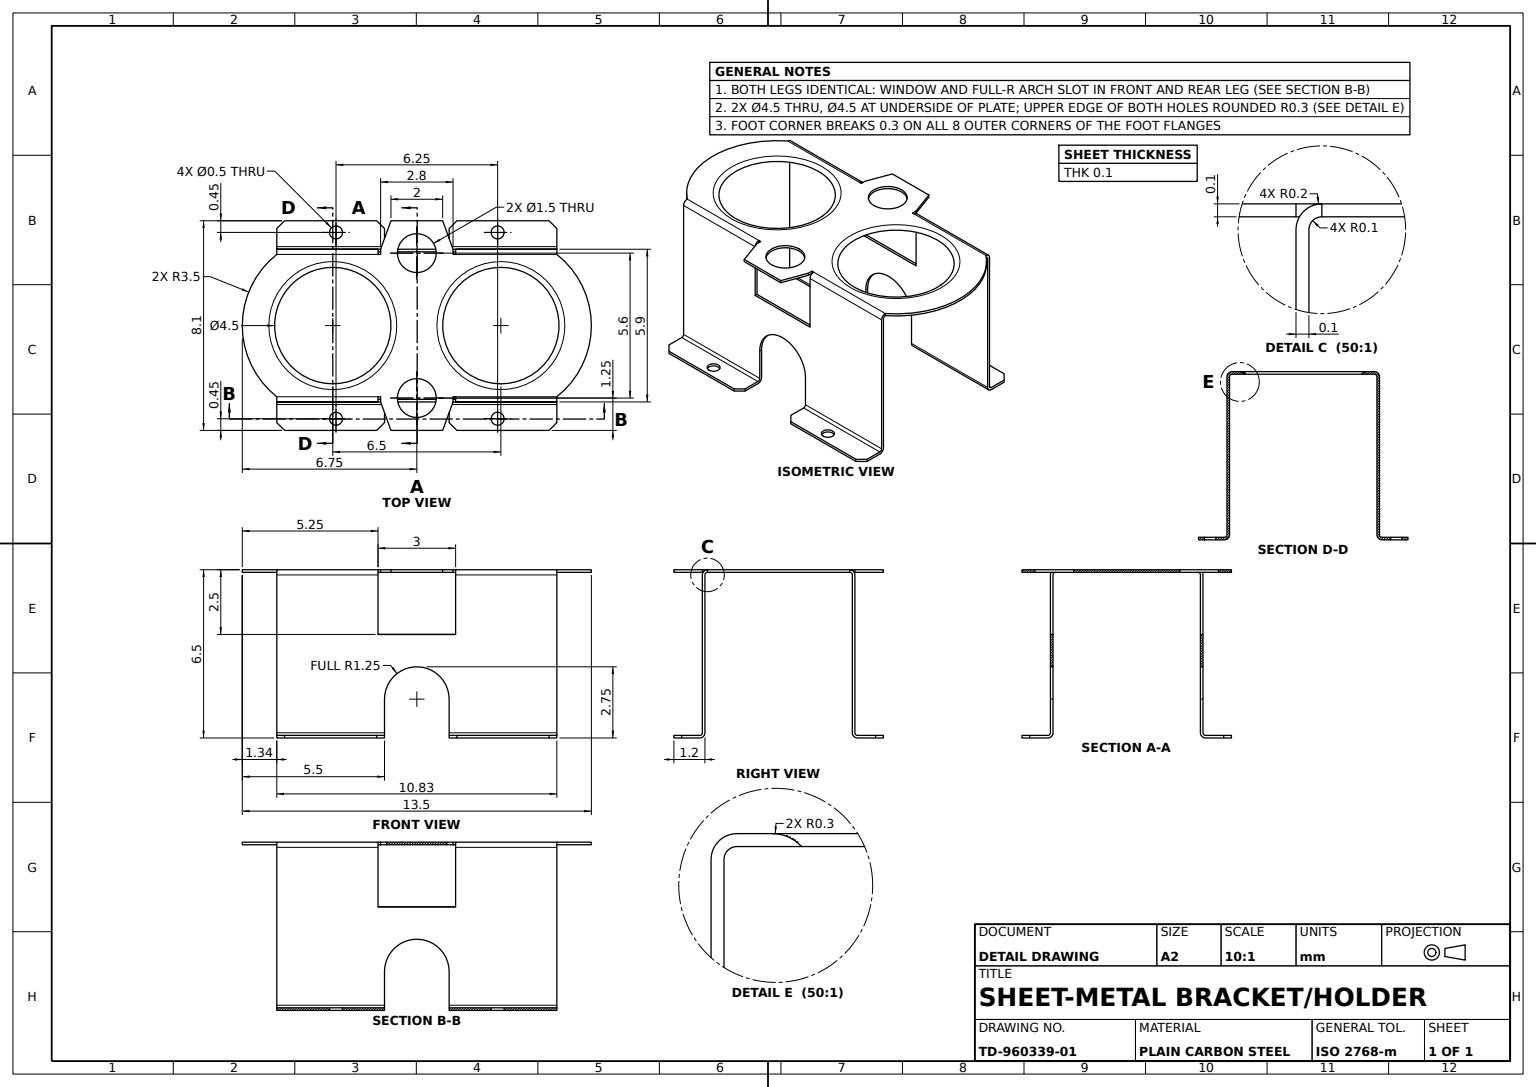
solid
v1 (-3.250103,0,-2.05)
v2 (-3.250103,0,-3.55)
e1 v1 v2 CIRCLE(AX(P(-3.250103,0,-2.8),D(0,-1,0),D(0,0,-1)),0.75)
v3 (-3.250103,-0.1,-2.05)
e2 v3 v1 LINE
v4 (-3.250103,-0.1,-3.55)
e3 v3 v4 CIRCLE(AX(P(-3.250103,-0.1,-2.8),D(0,-1,0),D(0,0,-1)),0.75)
e4 v4 v2 LINE
face CYL(AX(P(-3.250103,-0.1,-2.8),D(0,1,0),D(0,0,1)),0.75) rev [-e1 -e2 e3 e4]
v5 (2.164897,-6.3,-2.85)
v6 (2.164897,-6.5,-3.05)
e5 v5 v6 CIRCLE(AX(P(2.164897,-6.3,-3.05),D(1,0,0),D(0,0,1)),0.2)
v7 (-2.000103,-6.3,-2.85)
e6 v7 v5 LINE
v8 (-2.000103,-6.5,-3.05)
e7 v7 v8 CIRCLE(AX(P(-2.000103,-6.3,-3.05),D(1,0,0),D(0,-1,0)),0.2)
e8 v8 v6 LINE
face CYL(AX(P(-8.665103,-6.3,-3.05),D(-1,0,0),D(0,-1,0)),0.2) [-e5 -e6 e7 e8]
v9 (-1.750103,-0.2,2.85)
v10 (-1.750103,-0.1,2.75)
e9 v9 v10 CIRCLE(AX(P(-1.750103,-0.2,2.75),D(-1,0,0),D(0,0,-1)),0.1)
v11 (2.164897,-0.1,2.75)
e10 v10 v11 LINE
v12 (2.164897,-0.2,2.85)
e11 v11 v12 CIRCLE(AX(P(2.164897,-0.2,2.75),D(1,0,0),D(0,0,1)),0.1)
e12 v12 v9 LINE
face CYL(AX(P(-8.665103,-0.2,2.75),D(-1,0,0),D(0,0,1)),0.1) rev [e9 e10 e11 e12]
v13 (-4.750103,-2.5,2.85)
v14 (-4.750103,-2.5,2.95)
e13 v13 v14 LINE
v15 (-1.750103,-2.5,2.95)
e14 v15 v14 LINE
v16 (-1.750103,-2.5,2.85)
e15 v16 v15 LINE
e16 v16 v13 LINE
face PLANE(AX(P(-1.750103,-2.5,2.95),D(0,-1,0),D(-1,0,0))) rev [e13 -e14 -e15 e16]
v17 (-0.125103,-6.5,3.85)
v18 (-0.125103,-6.4,3.85)
e17 v17 v18 LINE
v19 (-0.125103,-6.4,3.35)
e18 v19 v18 CIRCLE(AX(P(-0.125103,-6.4,3.6),D(0,-1,0),D(0,0,1)),0.25)
v20 (-0.125103,-6.5,3.35)
e19 v20 v19 LINE
e20 v20 v17 CIRCLE(AX(P(-0.125103,-6.5,3.6),D(0,-1,0),D(0,0,1)),0.25)
face CYL(AX(P(-0.125103,-6.5,3.6),D(0,1,0),D(0,0,1)),0.25) rev [e17 -e18 -e19 e20]
v21 (-1.750103,-2.5,-2.85)
v22 (-1.750103,-2.5,-2.95)
e21 v21 v22 LINE
v23 (-4.750103,-2.5,-2.95)
e22 v23 v22 LINE
v24 (-4.750103,-2.5,-2.85)
e23 v24 v23 LINE
e24 v24 v21 LINE
face PLANE(AX(P(-4.750103,-2.5,-2.95),D(0,-1,0),D(1,0,0))) rev [e21 -e22 -e23 e24]
v25 (-2.000103,-6.5,3.05)
v26 (-2.000103,-6.3,2.85)
e25 v25 v26 CIRCLE(AX(P(-2.000103,-6.3,3.05),D(1,0,0),D(0,-1,0)),0.2)
v27 (-2.000103,-6.4,3.05)
e26 v27 v25 LINE
v28 (-2.000103,-6.3,2.95)
e27 v27 v28 CIRCLE(AX(P(-2.000103,-6.3,3.05),D(1,0,0),D(0,-1,0)),0.1)
e28 v26 v28 LINE
face PLANE(AX(P(-2.000103,-5,-4.05),D(-1,0,0),D(0,-1,0))) [-e25 -e26 e27 -e28]
v29 (2.164897,-6.4,3.75)
v30 (2.164897,-6.5,3.75)
e29 v29 v30 LINE
v31 (1.864897,-6.4,4.05)
e30 v31 v29 LINE
v32 (1.864897,-6.5,4.05)
e31 v32 v31 LINE
e32 v30 v32 LINE
face PLANE(AX(P(1.864897,-6.5,4.05),D(-0.707106781,0,-0.707106781),D(0,1,0))) rev [-e29 -e30 -e31 -e32]
v33 (-1.750103,-0.2,-2.85)
v34 (2.164897,-0.2,-2.85)
e33 v33 v34 LINE
v35 (2.164897,-0.1,-2.75)
e34 v34 v35 CIRCLE(AX(P(2.164897,-0.2,-2.75),D(1,0,0),D(0,0,-1)),0.1)
v36 (-1.750103,-0.1,-2.75)
e35 v35 v36 LINE
e36 v36 v33 CIRCLE(AX(P(-1.750103,-0.2,-2.75),D(-1,0,0),D(0,0,-1)),0.1)
face CYL(AX(P(2.164897,-0.2,-2.75),D(1,0,0),D(0,0,-1)),0.1) rev [e33 e34 e35 e36]
v37 (-1.850103,-0.1,-2.75)
v38 (-1.850103,0,-2.75)
e37 v37 v38 LINE
v39 (-1.750103,0,-2.75)
e38 v39 v38 LINE
e39 v36 v39 LINE
e40 v36 v37 LINE
face PLANE(AX(P(-1.750103,0,-2.75),D(0,0,1),D(-1,0,0))) rev [e37 -e38 -e39 e40]
v40 (-4.750103,-0.1,2.75)
v41 (-4.750103,-0.2,2.85)
e41 v40 v41 CIRCLE(AX(P(-4.750103,-0.2,2.75),D(1,0,0),D(0,0,1)),0.1)
v42 (-4.750103,0,2.75)
e42 v40 v42 LINE
v43 (-4.750103,-0.2,2.95)
e43 v42 v43 CIRCLE(AX(P(-4.750103,-0.2,2.75),D(1,0,0),D(0,0,1)),0.2)
e44 v14 v43 LINE
e45 v13 v41 LINE
face PLANE(AX(P(-4.750103,-0.2,2.75),D(-1,0,0),D(0,0,1))) rev [-e41 e42 e43 -e44 -e13 e45]
v44 (-8.665103,-6.5,3.75)
v45 (-8.665103,-6.4,3.75)
e46 v44 v45 LINE
v46 (-8.665103,-6.4,3.05)
e47 v45 v46 LINE
v47 (-8.665103,-6.5,3.05)
e48 v46 v47 LINE
e49 v44 v47 LINE
face PLANE(AX(P(-8.665103,-6.5,2.95),D(1,0,0),D(0,0,-1))) rev [e46 e47 e48 -e49]
v48 (-8.665103,-6.5,-3.05)
v49 (-4.500103,-6.5,-3.05)
e50 v48 v49 LINE
v50 (-4.500103,-6.3,-2.85)
e51 v49 v50 CIRCLE(AX(P(-4.500103,-6.3,-3.05),D(-1,0,0),D(0,1,0)),0.2)
v51 (-8.665103,-6.3,-2.85)
e52 v51 v50 LINE
e53 v48 v51 CIRCLE(AX(P(-8.665103,-6.3,-3.05),D(-1,0,0),D(0,0,1)),0.2)
face CYL(AX(P(-8.665103,-6.3,-3.05),D(-1,0,0),D(0,-1,0)),0.2) [e50 e51 -e52 -e53]
v52 (-4.250103,0,4.05)
v53 (-2.250103,0,4.05)
e54 v52 v53 LINE
v54 (-4.250103,-0.1,4.05)
e55 v54 v52 LINE
v55 (-2.250103,-0.1,4.05)
e56 v54 v55 LINE
e57 v55 v53 LINE
face PLANE(AX(P(-2.250103,-0.1,4.05),D(0,0,1),D(1,0,0))) [-e54 -e55 e56 e57]
v56 (-8.665103,-0.2,2.95)
v57 (-8.665103,-6.3,2.95)
e58 v56 v57 LINE
v58 (-4.500103,-6.3,2.95)
e59 v58 v57 LINE
v59 (-4.500103,-5,2.95)
e60 v59 v58 LINE
v60 (-2.000103,-5,2.95)
e61 v60 v59 CIRCLE(AX(P(-3.250103,-5,2.95),D(0,0,1),D(0,1,0)),1.25)
e62 v28 v60 LINE
v61 (2.164897,-6.3,2.95)
e63 v61 v28 LINE
v62 (2.164897,-0.2,2.95)
e64 v61 v62 LINE
v63 (-1.750103,-0.2,2.95)
e65 v63 v62 LINE
e66 v15 v63 LINE
e67 v56 v43 LINE
face PLANE(AX(P(0,0,2.95),D(0,0,-1),D(0,1,0))) rev [e58 -e59 -e60 -e61 -e62 -e63 e64 -e65 -e66 e14 e44 -e67]
v64 (-2.000103,-5,2.85)
e68 v64 v60 LINE
e69 v26 v64 LINE
face PLANE(AX(P(-2.000103,-5,-4.05),D(-1,0,0),D(0,-1,0))) [-e68 -e69 e28 e62]
v65 (-4.500103,-6.4,3.05)
e70 v58 v65 CIRCLE(AX(P(-4.500103,-6.3,3.05),D(-1,0,0),D(0,1,0)),0.1)
e71 v57 v46 CIRCLE(AX(P(-8.665103,-6.3,3.05),D(-1,0,0),D(0,0,-1)),0.1)
e72 v46 v65 LINE
face CYL(AX(P(2.164897,-6.3,3.05),D(1,0,0),D(0,-1,0)),0.1) rev [-e70 e59 e71 e72]
v66 (2.164897,-6.4,3.05)
e73 v66 v29 LINE
v67 (2.164897,-6.5,3.05)
e74 v67 v30 LINE
e75 v66 v67 LINE
face PLANE(AX(P(2.164897,-6.5,4.05),D(-1,0,0),D(0,0,1))) rev [e73 e29 -e74 -e75]
v68 (-2.000103,-6.4,-3.05)
e76 v8 v68 LINE
v69 (-2.000103,-6.4,-3.75)
e77 v69 v68 LINE
v70 (-2.000103,-6.5,-3.75)
e78 v69 v70 LINE
e79 v70 v8 LINE
face PLANE(AX(P(-2.000103,-5,-4.05),D(-1,0,0),D(0,-1,0))) [e76 -e77 e78 e79]
e80 v9 v16 LINE
v71 (-1.750103,0,2.75)
e81 v63 v71 CIRCLE(AX(P(-1.750103,-0.2,2.75),D(-1,0,0),D(0,0,1)),0.2)
e82 v10 v71 LINE
face PLANE(AX(P(-1.750103,-0.2,2.75),D(1,0,0),D(0,0,-1))) rev [e80 e15 e66 e81 -e82 -e9]
v72 (-4.500103,-6.4,-3.75)
v73 (-4.800103,-6.4,-4.05)
e83 v72 v73 LINE
v74 (-4.500103,-6.5,-3.75)
e84 v74 v72 LINE
v75 (-4.800103,-6.5,-4.05)
e85 v75 v74 LINE
e86 v73 v75 LINE
face PLANE(AX(P(-4.500103,-6.5,-3.75),D(0.707106781,0,-0.707106781),D(0,-1,0))) [-e83 -e84 -e85 -e86]
v76 (-1.850103,-0.1,-2.95)
v77 (-1.850103,0,-2.95)
e87 v76 v77 LINE
e88 v77 v38 LINE
e89 v76 v37 LINE
face PLANE(AX(P(-1.850103,-0.1,-2.95),D(-1,0,0),D(0,0,1))) rev [e87 e88 -e37 -e89]
v78 (-6.375103,-6.5,-3.35)
v79 (-6.375103,-6.5,-3.85)
e90 v78 v79 CIRCLE(AX(P(-6.375103,-6.5,-3.6),D(0,1,0),D(0,0,1)),0.25)
v80 (-6.375103,-6.4,-3.35)
e91 v78 v80 LINE
v81 (-6.375103,-6.4,-3.85)
e92 v80 v81 CIRCLE(AX(P(-6.375103,-6.4,-3.6),D(0,1,0),D(0,0,1)),0.25)
e93 v79 v81 LINE
face CYL(AX(P(-6.375103,-6.5,-3.6),D(0,1,0),D(0,0,1)),0.25) rev [-e90 e91 e92 -e93]
v82 (-8.665103,-0.2,2.85)
v83 (-8.665103,-6.3,2.85)
e94 v82 v83 LINE
e95 v57 v83 LINE
e96 v82 v56 LINE
face PLANE(AX(P(-8.665103,-6.5,2.95),D(1,0,0),D(0,0,-1))) rev [e94 -e95 -e58 -e96]
v84 (2.164897,-6.3,2.85)
e97 v67 v84 CIRCLE(AX(P(2.164897,-6.3,3.05),D(1,0,0),D(0,0,-1)),0.2)
e98 v61 v84 LINE
e99 v66 v61 CIRCLE(AX(P(2.164897,-6.3,3.05),D(1,0,0),D(0,0,-1)),0.1)
face PLANE(AX(P(2.164897,-6.3,3.05),D(-1,0,0),D(0,0,1))) rev [e75 e97 -e98 -e99]
v85 (-3.250103,0,2.05)
v86 (-3.250103,0,3.55)
e100 v85 v86 CIRCLE(AX(P(-3.250103,0,2.8),D(0,1,0),D(0,0,1)),0.75)
v87 (-3.250103,-0.1,3.55)
e101 v87 v86 LINE
v88 (-3.250103,-0.1,2.05)
e102 v88 v87 CIRCLE(AX(P(-3.250103,-0.1,2.8),D(0,1,0),D(0,0,1)),0.75)
e103 v88 v85 LINE
face CYL(AX(P(-3.250103,-0.1,2.8),D(0,1,0),D(0,0,1)),0.75) rev [e100 -e101 -e102 e103]
v89 (-2.000103,-6.3,-2.95)
e104 v89 v7 LINE
e105 v89 v68 CIRCLE(AX(P(-2.000103,-6.3,-3.05),D(1,0,0),D(0,-1,0)),0.1)
face PLANE(AX(P(-2.000103,-5,-4.05),D(-1,0,0),D(0,-1,0))) [-e76 -e7 -e104 e105]
e106 v79 v78 CIRCLE(AX(P(-6.375103,-6.5,-3.6),D(0,1,0),D(0,0,1)),0.25)
e107 v81 v80 CIRCLE(AX(P(-6.375103,-6.4,-3.6),D(0,1,0),D(0,0,1)),0.25)
face CYL(AX(P(-6.375103,-6.5,-3.6),D(0,1,0),D(0,0,1)),0.25) rev [-e106 e93 e107 -e91]
v90 (-4.750103,-0.2,-2.95)
v91 (-4.750103,0,-2.75)
e108 v90 v91 CIRCLE(AX(P(-4.750103,-0.2,-2.75),D(1,0,0),D(0,0,-1)),0.2)
v92 (-8.665103,-0.2,-2.95)
e109 v90 v92 LINE
v93 (-8.665103,0,-2.75)
e110 v93 v92 CIRCLE(AX(P(-8.665103,-0.2,-2.75),D(-1,0,0),D(0,0,-1)),0.2)
e111 v91 v93 LINE
face CYL(AX(P(2.164897,-0.2,-2.75),D(1,0,0),D(0,0,-1)),0.2) [-e108 e109 -e110 -e111]
v94 (2.164897,0,2.75)
e112 v11 v94 LINE
e113 v11 v35 CIRCLE(AX(P(0,-0.1,0),D(0,1,0),D(0,0,-1)),3.499897)
v95 (2.164897,0,-2.75)
e114 v35 v95 LINE
e115 v94 v95 CIRCLE(AX(P(0,0,0),D(0,1,0),D(0,0,-1)),3.499897)
face CYL(AX(P(0,-0.1,0),D(0,1,0),D(0,0,1)),3.499897) [-e112 e113 e114 -e115]
v96 (-4.500103,-6.5,3.05)
e116 v96 v65 LINE
v97 (-4.500103,-6.3,2.85)
e117 v97 v96 CIRCLE(AX(P(-4.500103,-6.3,3.05),D(-1,0,0),D(0,1,0)),0.2)
e118 v58 v97 LINE
face PLANE(AX(P(-4.500103,-6.5,-4.05),D(1,0,0),D(0,1,0))) [e70 -e116 -e117 -e118]
v98 (-8.665103,-6.3,-2.95)
v99 (-4.500103,-6.3,-2.95)
e119 v98 v99 LINE
e120 v98 v92 LINE
e121 v23 v90 LINE
v100 (-1.750103,-0.2,-2.95)
e122 v22 v100 LINE
v101 (2.164897,-0.2,-2.95)
e123 v101 v100 LINE
v102 (2.164897,-6.3,-2.95)
e124 v101 v102 LINE
e125 v89 v102 LINE
v103 (-2.000103,-5,-2.95)
e126 v103 v89 LINE
v104 (-4.500103,-5,-2.95)
e127 v104 v103 CIRCLE(AX(P(-3.250103,-5,-2.95),D(0,0,-1),D(0,-1,0)),1.25)
e128 v99 v104 LINE
face PLANE(AX(P(0,0,-2.95),D(0,0,1),D(0,-1,0))) rev [-e119 e120 -e109 -e121 e22 e122 -e123 e124 -e125 -e126 -e127 -e128]
e129 v39 v100 CIRCLE(AX(P(-1.750103,-0.2,-2.75),D(-1,0,0),D(0,0,-1)),0.2)
e130 v95 v39 LINE
e131 v101 v95 CIRCLE(AX(P(2.164897,-0.2,-2.75),D(1,0,0),D(0,0,-1)),0.2)
face CYL(AX(P(2.164897,-0.2,-2.75),D(1,0,0),D(0,0,-1)),0.2) [e123 -e129 -e130 -e131]
v105 (-4.500103,-6.4,-3.05)
v106 (-8.665103,-6.4,-3.05)
e132 v105 v106 LINE
e133 v106 v98 CIRCLE(AX(P(-8.665103,-6.3,-3.05),D(-1,0,0),D(0,0,1)),0.1)
e134 v105 v99 CIRCLE(AX(P(-4.500103,-6.3,-3.05),D(-1,0,0),D(0,1,0)),0.1)
face CYL(AX(P(-8.665103,-6.3,-3.05),D(-1,0,0),D(0,-1,0)),0.1) rev [e132 e133 e119 -e134]
v107 (-4.650103,-0.1,2.75)
v108 (-4.650103,-0.1,2.95)
e135 v107 v108 LINE
v109 (-4.650103,0,2.95)
e136 v108 v109 LINE
v110 (-4.650103,0,2.75)
e137 v110 v109 LINE
e138 v107 v110 LINE
face PLANE(AX(P(-4.650103,-0.1,2.95),D(-1,0,0),D(0,0,1))) [e135 e136 -e137 -e138]
e139 v21 v33 LINE
face PLANE(AX(P(-1.750103,-0.2,-2.75),D(1,0,0),D(0,0,-1))) rev [-e36 e39 e129 -e122 -e21 e139]
e140 v67 v25 LINE
v111 (-1.700103,-6.5,4.05)
e141 v32 v111 LINE
v112 (-2.000103,-6.5,3.75)
e142 v111 v112 LINE
e143 v25 v112 LINE
e144 v17 v20 CIRCLE(AX(P(-0.125103,-6.5,3.6),D(0,-1,0),D(0,0,1)),0.25)
face PLANE(AX(P(0,-6.5,0),D(0,1,0),D(0,0,1))) rev [-e140 e74 e32 e141 e142 -e143] [-e144 -e20]
v113 (-1.700103,-6.4,4.05)
e145 v113 v111 LINE
e146 v31 v113 LINE
face PLANE(AX(P(-8.665103,-6.5,4.05),D(0,0,-1),D(0,1,0))) rev [e145 -e141 e31 e146]
e147 v34 v101 LINE
e148 v34 v5 LINE
e149 v102 v5 LINE
face PLANE(AX(P(2.164897,-6.5,-2.95),D(-1,0,0),D(0,0,1))) rev [-e147 e148 -e149 -e124]
v114 (2.164897,-6.4,-3.05)
e150 v114 v6 LINE
e151 v102 v114 CIRCLE(AX(P(2.164897,-6.3,-3.05),D(1,0,0),D(0,0,1)),0.1)
face PLANE(AX(P(2.164897,-6.3,-3.05),D(1,0,0),D(0,0,-1))) [e5 -e150 -e151 e149]
v115 (-4.650103,0,-2.95)
v116 (-4.250103,0,-4.05)
e152 v115 v116 LINE
v117 (-4.250103,-0.1,-4.05)
e153 v117 v116 LINE
v118 (-4.650103,-0.1,-2.95)
e154 v118 v117 LINE
e155 v118 v115 LINE
face PLANE(AX(P(-4.250103,-0.1,-4.05),D(0.939793423,0,0.341743063),D(0.341743063,0,-0.939793423))) rev [e152 -e153 -e154 e155]
v119 (-8.665103,0,2.75)
e156 v56 v119 CIRCLE(AX(P(-8.665103,-0.2,2.75),D(-1,0,0),D(0,0,1)),0.2)
e157 v119 v42 LINE
face CYL(AX(P(-8.665103,-0.2,2.75),D(-1,0,0),D(0,0,1)),0.2) [-e156 e67 -e43 -e157]
v120 (-6.375103,-6.4,3.85)
v121 (-6.375103,-6.4,3.35)
e158 v120 v121 CIRCLE(AX(P(-6.375103,-6.4,3.6),D(0,-1,0),D(0,0,-1)),0.25)
e159 v121 v120 CIRCLE(AX(P(-6.375103,-6.4,3.6),D(0,-1,0),D(0,0,-1)),0.25)
v122 (-4.800103,-6.4,4.05)
v123 (-8.365103,-6.4,4.05)
e160 v122 v123 LINE
v124 (-4.500103,-6.4,3.75)
e161 v122 v124 LINE
e162 v124 v65 LINE
e163 v45 v123 LINE
face PLANE(AX(P(0,-6.4,0),D(0,1,0),D(0,0,1))) [e158 e159] [-e160 e161 e162 -e72 -e47 e163]
v125 (-1.850103,0,2.75)
e164 v125 v71 LINE
v126 (-1.850103,-0.1,2.75)
e165 v126 v125 LINE
e166 v126 v10 LINE
face PLANE(AX(P(-4.750103,0,2.75),D(0,0,-1),D(1,0,0))) rev [e82 -e164 -e165 e166]
v127 (-4.500103,-6.5,3.75)
e167 v124 v127 LINE
v128 (-4.800103,-6.5,4.05)
e168 v128 v122 LINE
e169 v127 v128 LINE
face PLANE(AX(P(-4.800103,-6.5,4.05),D(0.707106781,0,0.707106781),D(0,-1,0))) [-e167 -e161 -e168 -e169]
v129 (-4.500103,-5,2.85)
e170 v129 v97 LINE
e171 v97 v83 LINE
e172 v41 v82 LINE
e173 v84 v12 LINE
e174 v84 v26 LINE
e175 v64 v129 CIRCLE(AX(P(-3.250103,-5,2.85),D(0,0,1),D(0,1,0)),1.25)
face PLANE(AX(P(0,0,2.85),D(0,0,-1),D(0,1,0))) [e170 e171 -e94 -e172 -e45 -e16 -e80 -e12 -e173 e174 e69 e175]
v130 (-2.250103,0,-4.05)
e176 v116 v130 LINE
v131 (-2.250103,-0.1,-4.05)
e177 v131 v130 LINE
e178 v117 v131 LINE
face PLANE(AX(P(-2.250103,-0.1,-4.05),D(0,0,1),D(1,0,0))) rev [e176 -e177 -e178 e153]
e179 v50 v99 LINE
e180 v105 v49 LINE
face PLANE(AX(P(-4.500103,-6.5,-4.05),D(1,0,0),D(0,1,0))) [e134 -e179 -e51 -e180]
e181 v2 v1 CIRCLE(AX(P(-3.250103,0,-2.8),D(0,-1,0),D(0,0,-1)),0.75)
e182 v4 v3 CIRCLE(AX(P(-3.250103,-0.1,-2.8),D(0,-1,0),D(0,0,-1)),0.75)
face CYL(AX(P(-3.250103,-0.1,-2.8),D(0,1,0),D(0,0,1)),0.75) rev [-e181 -e4 e182 e2]
v132 (-8.665103,-6.4,-3.75)
e183 v106 v132 LINE
e184 v105 v72 LINE
v133 (-8.365103,-6.4,-4.05)
e185 v133 v73 LINE
e186 v133 v132 LINE
face PLANE(AX(P(0,-6.4,0),D(0,1,0),D(0,0,1))) [-e92 -e107] [-e183 -e132 e184 e83 -e185 e186]
v134 (-8.365103,-6.5,4.05)
e187 v123 v134 LINE
e188 v134 v44 LINE
face PLANE(AX(P(-8.665103,-6.5,3.75),D(0.707106781,0,-0.707106781),D(0,1,0))) rev [-e187 -e163 -e46 -e188]
e189 v74 v49 LINE
face PLANE(AX(P(-4.500103,-6.5,-4.05),D(1,0,0),D(0,1,0))) [-e189 e84 -e184 e180]
v135 (-1.850103,0,2.95)
e190 v53 v135 LINE
v136 (-1.850103,-0.1,2.95)
e191 v55 v136 LINE
e192 v136 v135 LINE
face PLANE(AX(P(-2.250103,-0.1,4.05),D(0.939793423,0,0.341743063),D(0.341743063,0,-0.939793423))) [-e190 -e57 e191 e192]
e193 v18 v19 CIRCLE(AX(P(-0.125103,-6.4,3.6),D(0,-1,0),D(0,0,1)),0.25)
face CYL(AX(P(-0.125103,-6.5,3.6),D(0,1,0),D(0,0,1)),0.25) rev [e144 e19 -e193 -e17]
v137 (-6.500206,-0.1,-2.25)
v138 (-6.500206,-0.1,2.25)
e194 v137 v138 CIRCLE(AX(P(-6.500206,-0.1,0),D(0,1,0),D(0,0,1)),2.25)
v139 (-6.500206,0,-2.473607)
e195 v137 v139 CIRCLE(AX(P(-6.500206,-0.3,-2.473607),D(-1,0,0),D(0,0,1)),0.3)
v140 (-6.500206,0,2.473607)
e196 v140 v139 CIRCLE(AX(P(-6.500206,0,0),D(0,-1,0),D(0,0,-1)),2.473607)
e197 v138 v140 CIRCLE(AX(P(-6.500206,-0.3,2.473607),D(1,0,0),D(0,0,-1)),0.3)
face TORUS(AX(P(-6.500206,-0.3,0),D(0,-1,0),D(0,0,-1)),2.473607,0.3) [-e194 e195 -e196 -e197]
e198 v27 v66 LINE
v141 (-2.000103,-6.4,3.75)
e199 v27 v141 LINE
e200 v141 v113 LINE
face PLANE(AX(P(0,-6.4,0),D(0,1,0),D(0,0,1))) [-e146 e30 -e73 -e198 e199 e200] [e193 e18]
v142 (2.164897,-6.4,-3.75)
v143 (1.864897,-6.4,-4.05)
e201 v142 v143 LINE
v144 (2.164897,-6.5,-3.75)
e202 v144 v142 LINE
v145 (1.864897,-6.5,-4.05)
e203 v145 v144 LINE
e204 v143 v145 LINE
face PLANE(AX(P(2.164897,-6.5,-3.75),D(-0.707106781,0,0.707106781),D(0,1,0))) rev [-e201 -e202 -e203 -e204]
v146 (-8.365103,-6.5,-4.05)
e205 v146 v75 LINE
e206 v146 v133 LINE
face PLANE(AX(P(2.164897,-6.5,-4.05),D(0,0,1),D(0,-1,0))) rev [e86 -e205 e206 e185]
v147 (-8.665103,-0.1,2.75)
e207 v147 v40 LINE
v148 (-8.665103,-0.1,-2.75)
e208 v148 v147 CIRCLE(AX(P(-6.500206,-0.1,0),D(0,1,0),D(0,0,1)),3.499897)
v149 (-4.750103,-0.1,-2.75)
e209 v149 v148 LINE
v150 (-4.650103,-0.1,-2.75)
e210 v150 v149 LINE
e211 v150 v118 LINE
e212 v131 v76 LINE
e213 v136 v126 LINE
e214 v108 v54 LINE
e215 v40 v107 LINE
e216 v138 v137 CIRCLE(AX(P(-6.500206,-0.1,0),D(0,1,0),D(0,0,1)),2.25)
e217 v87 v88 CIRCLE(AX(P(-3.250103,-0.1,2.8),D(0,1,0),D(0,0,1)),0.75)
v151 (0,-0.1,-2.25)
v152 (0,-0.1,2.25)
e218 v151 v152 CIRCLE(AX(P(0,-0.1,0),D(0,1,0),D(0,0,1)),2.25)
e219 v152 v151 CIRCLE(AX(P(0,-0.1,0),D(0,1,0),D(0,0,1)),2.25)
face PLANE(AX(P(0,-0.1,0),D(0,-1,0),D(0,0,-1))) [-e207 -e208 -e209 -e210 e211 e154 e178 e212 e89 -e40 -e35 -e113 -e10 -e166 -e213 -e191 -e56 -e214 -e135 -e215] [-e182 -e3] [e216 e194] [e102 e217] [e218 e219]
e220 v106 v48 LINE
v153 (-8.665103,-6.5,-3.75)
e221 v132 v153 LINE
e222 v48 v153 LINE
face PLANE(AX(P(-8.665103,-6.5,-4.05),D(1,0,0),D(0,0,-1))) rev [-e220 e183 e221 -e222]
e223 v112 v141 LINE
face PLANE(AX(P(-2.000103,-5,-4.05),D(-1,0,0),D(0,-1,0))) [e223 -e199 e26 e143]
e224 v142 v114 LINE
e225 v144 v6 LINE
face PLANE(AX(P(2.164897,-6.5,-2.95),D(-1,0,0),D(0,0,1))) rev [e202 e224 e150 -e225]
e226 v153 v146 LINE
face PLANE(AX(P(-8.365103,-6.5,-4.05),D(0.707106781,0,0.707106781),D(0,1,0))) rev [-e226 -e221 -e186 -e206]
v154 (-1.700103,-6.5,-4.05)
v155 (-1.700103,-6.4,-4.05)
e227 v154 v155 LINE
e228 v70 v154 LINE
e229 v155 v69 LINE
face PLANE(AX(P(-2.000103,-5,-3.75),D(-0.707106781,0,-0.707106781),D(0,1,0))) [-e227 -e228 -e78 -e229]
v156 (0,0,-2.473607)
e230 v151 v156 CIRCLE(AX(P(0,-0.3,-2.473607),D(-1,0,0),D(0,0,1)),0.3)
v157 (0,0,2.473607)
e231 v157 v156 CIRCLE(AX(P(0,0,0),D(0,-1,0),D(0,0,-1)),2.473607)
e232 v152 v157 CIRCLE(AX(P(0,-0.3,2.473607),D(1,0,0),D(0,0,-1)),0.3)
face TORUS(AX(P(0,-0.3,0),D(0,-1,0),D(0,0,-1)),2.473607,0.3) [-e218 e230 -e231 -e232]
v158 (-0.125103,-6.5,-3.85)
v159 (-0.125103,-6.5,-3.35)
e233 v158 v159 CIRCLE(AX(P(-0.125103,-6.5,-3.6),D(0,1,0),D(0,0,-1)),0.25)
e234 v159 v158 CIRCLE(AX(P(-0.125103,-6.5,-3.6),D(0,1,0),D(0,0,-1)),0.25)
e235 v154 v145 LINE
face PLANE(AX(P(0,-6.5,0),D(0,1,0),D(0,0,1))) rev [e233 e234] [e228 e235 e203 e225 -e8 -e79]
v160 (-4.500103,-5,-2.85)
e236 v104 v160 LINE
e237 v50 v160 LINE
face PLANE(AX(P(-4.500103,-6.5,-4.05),D(1,0,0),D(0,1,0))) [e236 -e237 e179 e128]
e238 v129 v59 LINE
face CYL(AX(P(-3.250103,-5,-4.05),D(0,0,1),D(1,0,0)),1.25) rev [e61 -e238 -e175 e68]
e239 v149 v91 LINE
v161 (-4.650103,0,-2.75)
e240 v161 v91 LINE
e241 v150 v161 LINE
face PLANE(AX(P(-1.750103,0,-2.75),D(0,0,1),D(-1,0,0))) rev [e239 -e240 -e241 e210]
e242 v147 v119 LINE
e243 v82 v147 CIRCLE(AX(P(-8.665103,-0.2,2.75),D(-1,0,0),D(0,0,1)),0.1)
face PLANE(AX(P(-8.665103,-0.2,2.75),D(1,0,0),D(0,0,-1))) rev [-e242 -e243 e96 e156]
e244 v156 v157 CIRCLE(AX(P(0,0,0),D(0,-1,0),D(0,0,-1)),2.473607)
face TORUS(AX(P(0,-0.3,0),D(0,-1,0),D(0,0,-1)),2.473607,0.3) [-e244 -e230 -e219 e232]
v162 (-4.750103,-0.2,-2.85)
e245 v162 v149 CIRCLE(AX(P(-4.750103,-0.2,-2.75),D(1,0,0),D(0,0,1)),0.1)
e246 v162 v24 LINE
face PLANE(AX(P(-4.750103,-0.2,-2.75),D(-1,0,0),D(0,0,1))) rev [e23 e121 e108 -e239 -e245 e246]
e247 v130 v77 LINE
face PLANE(AX(P(-2.250103,-0.1,-4.05),D(-0.939793423,0,0.341743063),D(0.341743063,0,0.939793423))) rev [e247 -e87 -e212 e177]
e248 v139 v140 CIRCLE(AX(P(-6.500206,0,0),D(0,-1,0),D(0,0,-1)),2.473607)
e249 v86 v85 CIRCLE(AX(P(-3.250103,0,2.8),D(0,1,0),D(0,0,1)),0.75)
e250 v161 v115 LINE
e251 v93 v119 CIRCLE(AX(P(-6.500206,0,0),D(0,1,0),D(0,0,1)),3.499897)
e252 v42 v110 LINE
e253 v109 v52 LINE
e254 v135 v125 LINE
e255 v71 v94 LINE
face PLANE(AX(P(0,0,0),D(0,-1,0),D(0,0,-1))) rev [e181 e1] [e231 e244] [e196 e248] [-e249 -e100] [-e152 -e250 e240 e111 e251 e157 e252 e137 e253 e54 e190 e254 e164 e255 e115 e130 e38 -e88 -e247 -e176]
face PLANE(AX(P(-4.750103,0,2.75),D(0,0,-1),D(1,0,0))) rev [-e252 -e42 e215 e138]
face PLANE(AX(P(-4.500103,-6.5,-4.05),D(1,0,0),D(0,1,0))) [-e170 e238 e60 e118]
e256 v98 v51 LINE
v163 (-8.665103,-0.2,-2.85)
e257 v51 v163 LINE
e258 v163 v92 LINE
face PLANE(AX(P(-8.665103,-0.1,-2.95),D(1,0,0),D(0,0,-1))) rev [-e120 e256 e257 e258]
v164 (-2.000103,-5,-2.85)
e259 v160 v164 CIRCLE(AX(P(-3.250103,-5,-2.85),D(0,0,-1),D(0,-1,0)),1.25)
e260 v103 v164 LINE
face CYL(AX(P(-3.250103,-5,-4.05),D(0,0,1),D(1,0,0)),1.25) rev [-e259 -e236 e127 e260]
e261 v96 v127 LINE
face PLANE(AX(P(-4.500103,-6.5,-4.05),D(1,0,0),D(0,1,0))) [-e261 e116 -e162 e167]
v165 (-6.375103,-6.5,3.85)
e262 v165 v120 LINE
v166 (-6.375103,-6.5,3.35)
e263 v165 v166 CIRCLE(AX(P(-6.375103,-6.5,3.6),D(0,-1,0),D(0,0,-1)),0.25)
e264 v166 v121 LINE
face CYL(AX(P(-6.375103,-6.5,3.6),D(0,1,0),D(0,0,1)),0.25) rev [-e158 -e262 e263 e264]
face CYL(AX(P(2.164897,-6.3,3.05),D(1,0,0),D(0,-1,0)),0.2) [-e174 -e97 e140 e25]
e265 v166 v165 CIRCLE(AX(P(-6.375103,-6.5,3.6),D(0,-1,0),D(0,0,-1)),0.25)
face CYL(AX(P(-6.375103,-6.5,3.6),D(0,1,0),D(0,0,1)),0.25) rev [-e159 -e264 e265 e262]
e266 v148 v163 CIRCLE(AX(P(-8.665103,-0.2,-2.75),D(-1,0,0),D(0,0,-1)),0.1)
e267 v148 v93 LINE
face PLANE(AX(P(-8.665103,-0.2,-2.75),D(-1,0,0),D(0,0,1))) [-e258 -e266 e267 e110]
face PLANE(AX(P(-1.850103,-0.1,2.95),D(1,0,0),D(0,0,-1))) [e213 e165 -e254 -e192]
e268 v163 v162 LINE
e269 v164 v7 LINE
face PLANE(AX(P(0,0,-2.85),D(0,0,1),D(0,-1,0))) [-e246 -e268 -e257 e52 e237 e259 e269 e6 -e148 -e33 -e139 -e24]
e270 v94 v62 CIRCLE(AX(P(2.164897,-0.2,2.75),D(1,0,0),D(0,0,1)),0.2)
e271 v12 v62 LINE
face PLANE(AX(P(2.164897,-0.2,2.75),D(1,0,0),D(0,0,-1))) [-e11 e112 e270 -e271]
e272 v128 v134 LINE
e273 v96 v47 LINE
face PLANE(AX(P(0,-6.5,0),D(0,1,0),D(0,0,1))) rev [e169 e272 e188 e49 -e273 e261] [-e263 -e265]
face CYL(AX(P(-3.250103,-0.1,2.8),D(0,1,0),D(0,0,1)),0.75) rev [-e217 e101 e249 -e103]
face PLANE(AX(P(-8.665103,-6.5,4.05),D(0,0,-1),D(0,1,0))) rev [-e272 e168 e160 e187]
face CYL(AX(P(-6.500206,-0.1,0),D(0,1,0),D(0,0,1)),3.499897) [-e267 e208 e242 -e251]
face CYL(AX(P(2.164897,-0.2,-2.75),D(1,0,0),D(0,0,-1)),0.1) rev [e268 e245 e209 e266]
v167 (-0.125103,-6.4,-3.85)
v168 (-0.125103,-6.4,-3.35)
e274 v167 v168 CIRCLE(AX(P(-0.125103,-6.4,-3.6),D(0,1,0),D(0,0,-1)),0.25)
e275 v159 v168 LINE
e276 v158 v167 LINE
face CYL(AX(P(-0.125103,-6.5,-3.6),D(0,1,0),D(0,0,1)),0.25) rev [e274 -e275 -e233 e276]
face PLANE(AX(P(-2.000103,-5,-4.05),D(-1,0,0),D(0,-1,0))) [-e269 -e260 e126 e104]
e277 v114 v68 LINE
face CYL(AX(P(-8.665103,-6.3,-3.05),D(-1,0,0),D(0,-1,0)),0.1) rev [-e105 e125 e151 e277]
face CYL(AX(P(2.164897,-6.3,3.05),D(1,0,0),D(0,-1,0)),0.1) rev [-e27 e198 e99 e63]
face PLANE(AX(P(-8.665103,-6.3,-3.05),D(1,0,0),D(0,0,-1))) rev [-e133 e220 e53 -e256]
e278 v155 v143 LINE
e279 v168 v167 CIRCLE(AX(P(-0.125103,-6.4,-3.6),D(0,1,0),D(0,0,-1)),0.25)
face PLANE(AX(P(0,-6.4,0),D(0,1,0),D(0,0,1))) [e77 -e277 -e224 e201 -e278 e229] [-e279 -e274]
face TORUS(AX(P(-6.500206,-0.3,0),D(0,-1,0),D(0,0,-1)),2.473607,0.3) [e197 -e248 -e195 -e216]
face PLANE(AX(P(-4.250103,-0.1,4.05),D(-0.939793423,0,0.341743063),D(0.341743063,0,0.939793423))) [-e136 e214 e55 -e253]
face PLANE(AX(P(2.164897,-6.5,-4.05),D(0,0,1),D(0,-1,0))) rev [e227 e278 e204 -e235]
face CYL(AX(P(-8.665103,-0.2,2.75),D(-1,0,0),D(0,0,1)),0.1) rev [e172 e243 e207 e41]
face PLANE(AX(P(-4.650103,-0.1,-2.95),D(1,0,0),D(0,0,-1))) rev [-e211 e241 e250 -e155]
face CYL(AX(P(-0.125103,-6.5,-3.6),D(0,1,0),D(0,0,1)),0.25) rev [-e234 e275 e279 -e276]
e280 v83 v47 CIRCLE(AX(P(-8.665103,-6.3,3.05),D(-1,0,0),D(0,0,-1)),0.2)
face PLANE(AX(P(-8.665103,-6.3,3.05),D(-1,0,0),D(0,0,1))) [e95 e280 -e48 -e71]
face PLANE(AX(P(-1.700103,-6.5,4.05),D(-0.707106781,0,0.707106781),D(0,1,0))) [-e200 -e223 -e142 -e145]
face PLANE(AX(P(2.164897,-0.1,2.95),D(-1,0,0),D(0,0,1))) rev [e271 -e64 e98 e173]
face PLANE(AX(P(2.164897,-0.2,-2.75),D(-1,0,0),D(0,0,1))) rev [-e114 -e34 e147 e131]
face CYL(AX(P(-8.665103,-0.2,2.75),D(-1,0,0),D(0,0,1)),0.2) [-e81 e65 -e270 -e255]
face CYL(AX(P(2.164897,-6.3,3.05),D(1,0,0),D(0,-1,0)),0.2) [-e171 e117 e273 -e280]
face PLANE(AX(P(0,-6.5,0),D(0,1,0),D(0,0,1))) rev [e90 e106] [e222 e226 e205 e85 e189 -e50]
